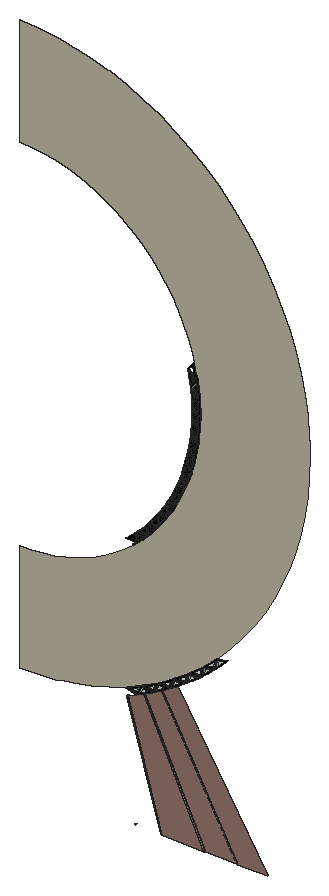
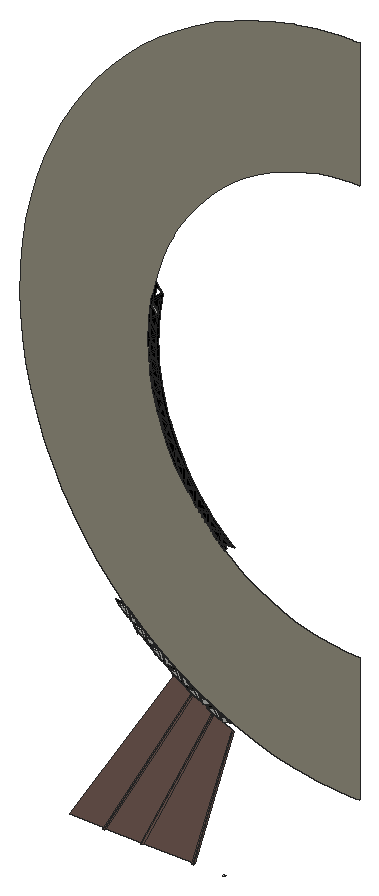
# SketchUp Ruby script. Lengths in inches.
U = 1.inch
M = Sketchup.active_model
def pt(a) = Geom::Point3d.new(a.map { |v| v * U })
def face(e, loops, mat)
  f = e.add_face(loops[0].map { |a| pt(a) })
  loops[1..].each { |l| e.add_face(l.map { |a| pt(a) }).erase! }
  f.material = f.back_material = mat if mat
  f
end
# faces: each face lists its corners as indices into pts; further lists are holes
def faces(e, pts, list, mat = nil) = list.each { |f| face(e, (f[0].is_a?(Array) ? f : [f]).map { |l| l.map { |i| pts[i] } }, mat) }
# xy, xz, yz: faces in a plane at the given z, y or x. An outline is a flat list of corners, or four numbers for a rectangle; further outlines are holes
def ring(l) = l.size == 4 ? [[l[0], l[1]], [l[2], l[1]], [l[2], l[3]], [l[0], l[3]]] : l.each_slice(2).to_a
def flat(e, list, mat, &to3) = list.each { |f| face(e, (f[0].is_a?(Array) ? f : [f]).map { |l| ring(l).map { |u, v| to3.(u, v) } }, mat) }
def xy(e, z, list, mat = nil) = flat(e, list, mat) { |x, y| [x, y, z] }
def xz(e, y, list, mat = nil) = flat(e, list, mat) { |x, z| [x, y, z] }
def yz(e, x, list, mat = nil) = flat(e, list, mat) { |y, z| [x, y, z] }
def lines(e, pts, list) = list.each { |a, b| e.add_line(pt(pts[a]), pt(pts[b])) }
# prism: a flat outline (further loops are holes) pulled along v
def prism(e, loops, v, mat = nil)
  f = face(e, loops, mat); d = Geom::Vector3d.new(v.map { |x| x * U })
  f.pushpull(f.normal.samedirection?(d) ? d.length : -d.length)
end
def box(e, o, s, mat = nil) = prism(e, [[o, [o[0] + s[0], o[1], o[2]], [o[0] + s[0], o[1] + s[1], o[2]], [o[0], o[1] + s[1], o[2]]]], [0, 0, s[2]], mat)
def at(x, y, z, deg = 0) = Geom::Transformation.translation(pt([x, y, z])) * Geom::Transformation.rotation(ORIGIN, Z_AXIS, deg.degrees)
def axes(o, x, y, z) = Geom::Transformation.new([*x, 0, *y, 0, *z, 0, *pt(o).to_a, 1])
def part(name) = M.definitions.add(name)
# library, detail: a bought-in or finely detailed component or shape, given as its bounding box
def library(name, o, s) = part(name).tap { |d| box(d.entities, o, s) }
def detail(e, o, s) = box(e.add_group.entities, o, s)
def put(e, d, t, mat = nil) = e.add_instance(d, t).tap { |i| i.material = mat if mat }
def group(e, t, mat = nil) = e.add_group.tap { |g| g.transformation = t; g.material = mat if mat }.entities
root = M.entities
M.materials.add("Tafisa-Terrarossa-PM780-4K").color = [148, 117, 107]
M.materials.add("Uniboard-L19-Putty-4K").color = [187, 181, 160]
M.materials.add("[Color M09]").color = [0, 0, 0]
xy(root,6.709,[[112.905,138,113.026,138.157],[115.672,138,115.795,138.157],[120.336,138,120.468,138.157]])
xy(root,22.994,[[118.808,138,119.552,138.157]])
xy(root,23.244,[[119.127,138,119.823,138.157]])
xy(root,33.737,[[112.411,138,113.165,138.125]],"[Color M09]")
xy(root,35.646,[[114.454,138,115.13,138.125]],"[Color M09]")
xy(root,35.892,[[114.604,138,115.342,138.157]],"[Color M09]")
xy(root,37.097,[[115.614,138,116.248,138.157]],"[Color M09]")
xy(root,37.343,[[115.741,138,116.358,138.157]],"[Color M09]")
xy(root,38.633,[[116.62,138,117.217,138.157]],"[Color M09]")
xy(root,38.879,[[116.715,138,117.293,138.157]],"[Color M09]")
xz(root,138,[[115.795,6.709,120.336,6.709,113.927,19.441,113.923,19.447,113.124,19.101,112.216,18.708],[120.468,6.709,123.753,6.709,115.795,20.393,114.914,19.943,114.032,19.494],[123.89,6.709,127.065,6.709,117.499,21.4,116.647,20.896,115.898,20.452,123.855,6.768]],"Tafisa-Terrarossa-PM780-4K")
xz(root,138,[[[113.124,19.101,113.73,20.136,111.955,19.367],[113.062,19.243,112.356,19.404,113.429,19.869]],[[113.124,19.101,113.923,19.447,114.032,19.494,114.914,19.943,113.73,20.136],[113.425,19.368,113.795,19.998,114.516,19.881,113.979,19.607]],[[114.914,19.943,115.454,21.014,113.73,20.136],[114.843,20.082,114.128,20.198,115.17,20.729]],[[114.914,19.943,115.795,20.393,115.898,20.452,116.647,20.896,115.454,21.014],[115.198,20.229,115.527,20.881,116.254,20.809,115.735,20.502]],[[116.647,20.896,117.119,21.999,115.454,21.014],[116.568,21.03,115.847,21.101,116.853,21.696]],
  [[116.647,20.896,117.499,21.4,117.597,21.466,118.317,21.956,117.119,21.999],[116.913,21.199,117.2,21.87,117.931,21.845,117.432,21.506]],[[118.317,21.956,118.704,23.076,117.119,21.999],[118.229,22.085,117.506,22.11,118.463,22.76]],[[118.317,21.956,119.136,22.512,119.229,22.586,119.918,23.119,118.762,23.119,118.719,23.086,118.704,23.076],[118.559,22.272,118.808,22.994,119.552,22.994,119.062,22.614]],[[118.762,23.119,119.918,23.119,120.248,24.272],[119.127,23.244,120.022,23.938,119.823,23.244]],[[119.918,23.119,120.7,23.725,120.789,23.803,121.442,24.38,120.248,24.272],[120.144,23.452,120.345,24.155,121.072,24.221,120.62,23.822]],
  [[120.248,24.272,121.442,24.38,121.699,25.551],[120.618,24.431,121.495,25.204,121.339,24.496]],[[121.442,24.38,122.184,25.034,122.884,25.734,121.699,25.551],[121.646,24.727,121.803,25.441,122.525,25.552,122.099,25.126]],[[112.052,33.614,113.301,33.614,113.203,34.599,112.336,33.835],[112.411,33.737,112.415,33.74,113.104,34.348,113.165,33.737]],[[113.301,33.614,113.753,34.013,114.331,34.591,113.203,34.599],[113.399,33.865,113.339,34.475,114.036,34.47,113.669,34.103]],[[114.331,34.591,114.331,35.769,114.019,35.415,113.203,34.599],[114.208,34.715,113.498,34.72,114.109,35.331,114.208,35.444]],
  [[114.331,34.591,114.605,34.865,115.402,35.769,114.331,35.769],[114.454,34.888,114.454,35.646,115.13,35.646,114.515,34.95]],[[114.331,35.769,115.402,35.769,115.491,35.884,115.491,37.194,114.783,36.282],[114.604,35.892,114.878,36.203,115.368,36.835,115.368,35.926,115.342,35.892]],[[115.491,35.884,116.141,36.722,116.48,37.22,115.509,37.22,115.491,37.194],[115.614,36.243,115.614,37.097,116.248,37.097,116.042,36.794]],[[115.509,37.22,116.48,37.22,116.499,38.756,116.14,38.15],[115.741,37.343,116.244,38.084,116.37,38.297,116.358,37.343]],[[116.48,37.22,116.819,37.719,117.432,38.756,116.499,38.756],[116.608,37.628,116.62,38.633,117.217,38.633,116.715,37.785]],
  [[116.499,38.756,117.432,38.756,117.252,40.173,116.728,39.144],[116.715,38.879,116.836,39.084,117.181,39.761,117.293,38.879]],[[117.432,38.756,117.979,39.83,118.371,40.735,117.252,40.173],[117.504,39.168,117.385,40.102,118.124,40.473,117.868,39.883]],[[117.252,40.173,118.371,40.735,117.906,41.776,117.711,41.233],[117.5,40.435,117.825,41.187,117.919,41.447,118.211,40.792]],[[118.371,40.735,118.458,40.937,118.867,42.071,118.911,42.225,117.906,41.776],[118.367,41.046,118.069,41.714,118.71,42]],[[117.906,41.776,118.911,42.225,118.424,43.428,118.102,42.319],[118.12,42.006,118.219,42.281,118.443,43.053,118.753,42.288]],
  [[118.911,42.225,119.203,43.228,119.334,43.816,118.424,43.428],[118.892,42.6,118.584,43.362,119.162,43.609,119.084,43.259]],[[118.424,43.428,119.334,43.816,118.69,44.641,118.676,44.555],[118.597,43.635,118.757,44.354,119.139,43.867]],[[119.334,43.816,119.466,44.405,119.605,45.287,118.69,44.641],[119.271,44.097,118.866,44.615,119.438,45.018,119.345,44.428]],[[118.69,44.641,119.605,45.287,118.911,46.271,118.857,45.696],[118.857,44.909,118.979,45.68,119.002,45.928,119.434,45.316]],[[119.605,45.287,119.654,45.595,119.768,46.795,118.911,46.271],[119.531,45.605,119.087,46.234,119.622,46.562,119.532,45.611]],
  [[118.911,46.271,119.768,46.795,118.984,47.423,118.966,46.846],[119.057,46.504,119.088,46.838,119.099,47.173,119.554,46.809]],[[119.768,46.795,119.806,48,118.984,47.423],[119.653,47.045,119.189,47.416,119.675,47.758]],[[118.984,47.423,119.806,48,118.984,48.577,119.002,48],[119.114,47.665,119.125,48,119.114,48.335,119.592,48]],[119.806,48,119.768,49.205,119.761,49.281,119.637,49.281,119.645,49.197,119.675,48.242,119.156,48.607,119.637,49.281,119.761,49.281,119.728,49.621,118.984,48.577],[[118.984,48.577,119.728,49.621,118.857,50.304,118.966,49.154],[119.095,48.945,119.088,49.162,119.006,50.031,119.56,49.597]],
  [[119.728,49.621,119.654,50.405,119.533,51.168,118.857,50.304],[119.579,49.895,119.03,50.325,119.456,50.87,119.532,50.389]],[[118.857,50.304,119.533,51.168,118.55,52.008,118.676,51.445],[118.934,50.602,118.797,51.468,118.751,51.675,119.364,51.151]],[[119.533,51.168,119.466,51.595,119.203,52.772,118.55,52.008],[119.36,51.478,118.724,52.022,119.136,52.505,119.345,51.572]]],"[Color M09]")
xz(root,138.125,[[112.411,33.737,113.165,33.737,113.104,34.348,112.415,33.74],[113.399,33.865,113.669,34.103,114.036,34.47,113.339,34.475],[114.208,34.715,114.208,35.444,114.109,35.331,113.498,34.72],[114.454,34.888,114.515,34.95,115.13,35.646,114.454,35.646]],"[Color M09]")
xz(root,138.157,[[113.062,19.243,113.429,19.869,112.356,19.404],[113.425,19.368,113.979,19.607,114.516,19.881,113.795,19.998],[114.843,20.082,115.17,20.729,114.128,20.198],[115.198,20.229,115.735,20.502,116.254,20.809,115.527,20.881],[116.568,21.03,116.853,21.696,115.847,21.101],
  [116.913,21.199,117.432,21.506,117.931,21.845,117.2,21.87],[118.229,22.085,118.463,22.76,117.506,22.11],[118.559,22.272,119.062,22.614,119.552,22.994,118.808,22.994],[119.127,23.244,119.823,23.244,120.022,23.938],[120.144,23.452,120.62,23.822,121.072,24.221,120.345,24.155],
  [120.618,24.431,121.339,24.496,121.495,25.204],[121.646,24.727,122.099,25.126,122.525,25.552,121.803,25.441]])
xz(root,138.157,[[115.672,6.709,115.795,6.709,112.216,18.708,112.104,18.668],[120.336,6.709,120.468,6.709,114.032,19.494,113.923,19.447,113.927,19.441],[123.753,6.709,123.89,6.709,123.855,6.768,115.898,20.452,115.795,20.393]],"Tafisa-Terrarossa-PM780-4K")
xz(root,138.157,[[100.618,17.205,100.931,17.214,101.585,17.235,102.552,17.265,104.478,17.447,105.433,17.599,106.389,17.75,108.277,18.172,110.134,18.712,111.955,19.367,113.73,20.136,115.454,21.014,117.119,21.999,118.704,23.076,118.719,23.086,118.762,23.119,120.248,24.272,121.699,25.551,123.067,26.919,124.346,28.37,125.532,29.899,126.619,31.499,127.604,33.164,128.483,34.888,128.867,35.776,129.251,36.663,129.906,38.484,130.446,40.342,130.868,42.23,131.171,44.14,131.353,46.066,131.413,48,131.373,49.281,131.353,49.934,131.171,51.86,130.868,53.77,130.446,55.658,129.906,57.516,129.251,59.337,128.483,61.112,127.604,62.836,126.619,64.501,125.532,66.101,124.346,67.63,123.067,69.081,121.699,70.449,120.248,71.728,118.719,72.914,117.119,74.001,115.454,74.986,113.73,75.864,111.955,76.633,110.134,77.288,109.87,77.365,108.277,77.828,106.612,78.2,106.389,78.25,105.433,78.401,104.478,78.553,102.552,78.735,101.327,78.773,101.236,78.776,101.221,78.776,100.618,78.795,100.618,67.1875,101.221,67.169,101.823,67.15,103.023,67.036,104.213,66.848,105.39,66.585,106.547,66.248,107.682,65.84,108.788,65.361,109.862,64.814,110.899,64.201,111.896,63.523,112.849,62.784,113.753,61.987,114.605,61.135,115.402,60.231,116.141,59.278,116.819,58.281,117.432,57.244,117.503,57.105,117.979,56.17,118.188,55.688,118.458,55.063,118.761,54.223,118.867,53.929,119.203,52.772,119.466,51.595,119.533,51.168,119.654,50.405,119.728,49.621,119.761,49.281,119.768,49.205,119.806,48,119.768,46.795,119.654,45.595,119.605,45.287,119.466,44.405,119.334,43.816,119.203,43.228,118.911,42.225,118.867,42.071,118.458,40.937,118.371,40.735,117.979,39.83,117.432,38.756,116.819,37.719,116.48,37.22,116.141,36.722,115.491,35.884,115.402,35.769,114.605,34.865,113.753,34.013,113.301,33.614,112.849,33.216,112.052,32.598,111.939,32.51,111.896,32.477,110.899,31.799,109.862,31.186,108.788,30.639,107.682,30.16,106.547,29.752,105.39,29.415,104.213,29.152,103.023,28.964,101.823,28.85,101.221,28.831,100.618,28.8125]],"Uniboard-L19-Putty-4K")
xz(root,138.157,[[114.604,35.892,115.342,35.892,115.368,35.926,115.368,36.835,114.878,36.203],[115.614,36.243,116.042,36.794,116.248,37.097,115.614,37.097],[115.741,37.343,116.358,37.343,116.37,38.297,116.244,38.084],[116.608,37.628,116.715,37.785,117.217,38.633,116.62,38.633],[116.715,38.879,117.293,38.879,117.181,39.761,116.836,39.084],
  [117.504,39.168,117.868,39.883,118.124,40.473,117.385,40.102],[117.5,40.435,118.211,40.792,117.919,41.447,117.825,41.187],[118.367,41.046,118.71,42,118.069,41.714],[118.12,42.006,118.753,42.288,118.443,43.053,118.219,42.281],[118.892,42.6,119.084,43.259,119.162,43.609,118.584,43.362],
  [118.597,43.635,119.139,43.867,118.757,44.354],[119.271,44.097,119.345,44.428,119.438,45.018,118.866,44.615],[118.857,44.909,119.434,45.316,119.002,45.928,118.979,45.68],[119.531,45.605,119.532,45.611,119.622,46.562,119.087,46.234],[119.057,46.504,119.554,46.809,119.099,47.173,119.088,46.838],
  [119.653,47.045,119.675,47.758,119.189,47.416],[119.114,47.665,119.592,48,119.114,48.335,119.125,48],[119.675,48.242,119.645,49.197,119.637,49.281,119.156,48.607],[119.095,48.945,119.56,49.597,119.006,50.031,119.088,49.162],[119.579,49.895,119.532,50.389,119.456,50.87,119.03,50.325],
  [118.934,50.602,119.364,51.151,118.751,51.675,118.797,51.468]],"[Color M09]")
yz(root,114.208,[[138,34.715,138.125,35.444]],"[Color M09]")
yz(root,114.454,[[138,34.888,138.125,35.646]],"[Color M09]")
yz(root,115.368,[[138,35.926,138.157,36.835]],"[Color M09]")
yz(root,115.614,[[138,36.243,138.157,37.097]],"[Color M09]")
p = [[112.104,138,18.668],[115.672,138,6.709],[115.672,138.157,6.709],[112.104,138.157,18.668],[115.795,138,6.709],[112.216,138,18.708],
  [112.216,138.157,18.708],[115.795,138.157,6.709],[113.927,138,19.441],[120.336,138,6.709],[120.336,138.157,6.709],[113.927,138.157,19.441],
  [120.468,138,6.709],[114.032,138,19.494],[114.032,138.157,19.494],[120.468,138.157,6.709],[115.795,138,20.393],[123.753,138,6.709],
  [123.753,138.157,6.709],[115.795,138.157,20.393],[123.855,138,6.768],[115.898,138,20.452],[115.898,138.157,20.452],[123.855,138.157,6.768],
  [112.356,138,19.404],[113.062,138,19.243],[113.062,138.157,19.243],[112.356,138.157,19.404],[113.429,138,19.869],[113.429,138.157,19.869],
  [111.955,138,19.367],[113.73,138,20.136],[113.73,138.157,20.136],[111.955,138.157,19.367],[113.795,138,19.998],[113.425,138,19.368],
  [113.425,138.157,19.368],[113.795,138.157,19.998],[113.979,138,19.607],[113.979,138.157,19.607],[113.923,138,19.447],[113.923,138.157,19.447],
  [114.516,138,19.881],[114.516,138.157,19.881],[115.454,138,21.014],[115.454,138.157,21.014],[114.128,138,20.198],[114.843,138,20.082],
  [114.843,138.157,20.082],[114.128,138.157,20.198],[115.17,138,20.729],[115.17,138.157,20.729],[115.527,138,20.881],[115.198,138,20.229],
  [115.198,138.157,20.229],[115.527,138.157,20.881],[115.735,138,20.502],[115.735,138.157,20.502],[116.254,138,20.809],[116.254,138.157,20.809],
  [117.119,138,21.999],[117.119,138.157,21.999],[115.847,138,21.101],[116.568,138,21.03],[116.568,138.157,21.03],[115.847,138.157,21.101],
  [116.853,138,21.696],[116.853,138.157,21.696],[117.2,138,21.87],[116.913,138,21.199],[116.913,138.157,21.199],[117.2,138.157,21.87],
  [117.432,138,21.506],[117.432,138.157,21.506],[117.597,138,21.466],[117.499,138,21.4],[117.499,138.157,21.4],[117.597,138.157,21.466],
  [117.931,138,21.845],[117.931,138.157,21.845],[117.598,138,21.464],[117.598,138.157,21.464],[118.704,138,23.076],[118.704,138.157,23.076],
  [117.506,138,22.11],[118.229,138,22.085],[118.229,138.157,22.085],[117.506,138.157,22.11],[118.463,138,22.76],[118.463,138.157,22.76],
  [118.808,138,22.994],[118.559,138,22.272],[118.559,138.157,22.272],[118.808,138.157,22.994],[119.062,138,22.614],[119.062,138.157,22.614],
  [119.229,138,22.586],[119.136,138,22.512],[119.136,138.157,22.512],[119.229,138.157,22.586],[119.552,138,22.994],[119.552,138.157,22.994],
  [118.719,138,23.086],[118.719,138.157,23.086],[118.762,138,23.119],[118.762,138.157,23.119],[120.248,138,24.272],[120.248,138.157,24.272],
  [120.022,138,23.938],[119.127,138,23.244],[119.127,138.157,23.244],[120.022,138.157,23.938],[119.823,138,23.244],[119.823,138.157,23.244],
  [120.345,138,24.155],[120.144,138,23.452],[120.144,138.157,23.452],[120.345,138.157,24.155],[120.62,138,23.822],[120.62,138.157,23.822],
  [120.789,138,23.803],[120.7,138,23.725],[120.7,138.157,23.725],[120.789,138.157,23.803],[121.072,138,24.221],[121.072,138.157,24.221],
  [121.699,138,25.551],[121.699,138.157,25.551],[120.618,138,24.431],[121.339,138,24.496],[121.339,138.157,24.496],[120.618,138.157,24.431],
  [121.495,138,25.204],[121.495,138.157,25.204],[121.803,138,25.441],[121.646,138,24.727],[121.646,138.157,24.727],[121.803,138.157,25.441],
  [122.099,138,25.126],[122.099,138.157,25.126],[122.525,138,25.552],[122.525,138.157,25.552],[113.301,138,33.614],[112.849,138,33.216],
  [112.849,138.157,33.216],[113.301,138.157,33.614],[112.77,138,33.311],[112.975,138,33.491],[112.975,138.125,33.491],[112.77,138.125,33.311],
  [113.753,138,34.013],[113.753,138.157,34.013],[113.104,138,34.348],[112.415,138,33.74],[112.415,138.125,33.74],[113.104,138.125,34.348],
  [113.165,138,33.737],[113.165,138.125,33.737],[112.336,138,33.835],[113.203,138,34.599],[113.203,138.157,34.599],[112.336,138.157,33.835],
  [113.339,138,34.475],[113.399,138,33.865],[113.399,138.125,33.865],[113.339,138.125,34.475],[113.669,138,34.103],[113.669,138.125,34.103],
  [114.331,138,34.591],[114.331,138.157,34.591],[114.036,138,34.47],[114.036,138.125,34.47],[114.019,138,35.415],[114.019,138.157,35.415],
  [114.605,138,34.865],[114.605,138.157,34.865],[114.109,138,35.331],[113.498,138,34.72],[113.498,138.125,34.72],[114.109,138.125,35.331],
  [114.208,138,34.715],[114.208,138.125,34.715],[114.454,138,34.888],[114.515,138,34.95],[114.515,138.125,34.95],[114.454,138.125,34.888],
  [115.13,138,35.646],[115.13,138.125,35.646],[115.402,138,35.769],[115.402,138.157,35.769],[114.208,138,35.444],[114.208,138.125,35.444],
  [114.331,138,35.769],[114.331,138.157,35.769],[114.783,138,36.282],[114.783,138.157,36.282],[115.491,138,35.884],[115.491,138.157,35.884],
  [114.878,138,36.203],[114.604,138,35.892],[114.604,138.157,35.892],[114.878,138.157,36.203],[115.342,138,35.892],[115.368,138,35.926],
  [115.368,138.157,35.926],[115.342,138.157,35.892],[116.141,138,36.722],[116.141,138.157,36.722],[115.368,138,36.835],[115.368,138.157,36.835],
  [115.614,138,36.243],[116.042,138,36.794],[116.042,138.157,36.794],[115.614,138.157,36.243],[115.491,138,37.194],[115.491,138.157,37.194],
  [116.48,138,37.22],[116.48,138.157,37.22],[116.248,138,37.097],[116.248,138.157,37.097],[115.509,138,37.22],[115.509,138.157,37.22],
  [116.14,138,38.15],[116.14,138.157,38.15],[116.819,138,37.719],[116.819,138.157,37.719],[116.244,138,38.084],[115.741,138,37.343],
  [115.741,138.157,37.343],[116.244,138.157,38.084],[116.358,138,37.343],[116.37,138,38.297],[116.37,138.157,38.297],[116.358,138.157,37.343],
  [116.62,138,38.633],[116.608,138,37.628],[116.608,138.157,37.628],[116.62,138.157,38.633],[116.715,138,37.785],[116.715,138.157,37.785],
  [117.432,138,38.756],[117.432,138.157,38.756],[117.217,138,38.633],[117.217,138.157,38.633],[116.499,138,38.756],[116.499,138.157,38.756],
  [116.728,138,39.144],[116.728,138.157,39.144],[117.979,138,39.83],[117.979,138.157,39.83],[116.836,138,39.084],[116.715,138,38.879],
  [116.715,138.157,38.879],[116.836,138.157,39.084],[117.293,138,38.879],[117.181,138,39.761],[117.181,138.157,39.761],[117.293,138.157,38.879],
  [117.252,138,40.173],[117.252,138.157,40.173],[117.385,138,40.102],[117.504,138,39.168],[117.504,138.157,39.168],[117.385,138.157,40.102],
  [117.868,138,39.883],[117.868,138.157,39.883],[118.371,138,40.735],[118.371,138.157,40.735],[118.124,138,40.473],[118.124,138.157,40.473],
  [117.711,138,41.233],[117.711,138.157,41.233],[117.825,138,41.187],[117.5,138,40.435],[117.5,138.157,40.435],[117.825,138.157,41.187],
  [118.211,138,40.792],[118.211,138.157,40.792],[118.458,138,40.937],[118.458,138.157,40.937],[117.919,138,41.447],[117.919,138.157,41.447],
  [118.867,138,42.071],[118.867,138.157,42.071],[118.069,138,41.714],[118.367,138,41.046],[118.367,138.157,41.046],[118.069,138.157,41.714],
  [118.71,138,42],[118.71,138.157,42],[117.906,138,41.776],[117.906,138.157,41.776],[118.102,138,42.319],[118.102,138.157,42.319],
  [118.219,138,42.281],[118.12,138,42.006],[118.12,138.157,42.006],[118.219,138.157,42.281],[118.753,138,42.288],[118.753,138.157,42.288],
  [118.911,138,42.225],[118.911,138.157,42.225],[119.203,138,43.228],[119.203,138.157,43.228],[118.424,138,43.428],[118.424,138.157,43.428],
  [118.443,138,43.053],[118.443,138.157,43.053],[118.584,138,43.362],[118.892,138,42.6],[118.892,138.157,42.6],[118.584,138.157,43.362],
  [119.084,138,43.259],[119.084,138.157,43.259],[119.334,138,43.816],[119.334,138.157,43.816],[119.162,138,43.609],[119.162,138.157,43.609],
  [118.676,138,44.555],[118.676,138.157,44.555],[118.757,138,44.354],[118.597,138,43.635],[118.597,138.157,43.635],[118.757,138.157,44.354],
  [119.139,138,43.867],[119.139,138.157,43.867],[119.466,138,44.405],[119.466,138.157,44.405],[118.866,138,44.615],[119.271,138,44.097],
  [119.271,138.157,44.097],[118.866,138.157,44.615],[119.345,138,44.428],[119.345,138.157,44.428],[119.438,138,45.018],[119.438,138.157,45.018],
  [119.605,138,45.287],[119.605,138.157,45.287],[118.69,138,44.641],[118.69,138.157,44.641],[118.857,138,45.696],[118.857,138.157,45.696],
  [118.979,138,45.68],[118.857,138,44.909],[118.857,138.157,44.909],[118.979,138.157,45.68],[119.434,138,45.316],[119.434,138.157,45.316],
  [119.002,138,45.928],[119.002,138.157,45.928],[119.654,138,45.595],[119.654,138.157,45.595],[119.087,138,46.234],[119.531,138,45.605],
  [119.531,138.157,45.605],[119.087,138.157,46.234],[119.532,138,45.611],[119.532,138.157,45.611],[119.622,138,46.562],[119.622,138.157,46.562],
  [119.768,138,46.795],[119.768,138.157,46.795],[118.911,138,46.271],[118.911,138.157,46.271],[118.966,138,46.846],[118.966,138.157,46.846],
  [119.088,138,46.838],[119.057,138,46.504],[119.057,138.157,46.504],[119.088,138.157,46.838],[119.554,138,46.809],[119.554,138.157,46.809],
  [118.984,138,47.423],[118.984,138.157,47.423],[119.099,138,47.173],[119.099,138.157,47.173],[119.806,138,48],[119.806,138.157,48],
  [119.189,138,47.416],[119.653,138,47.045],[119.653,138.157,47.045],[119.189,138.157,47.416],[119.675,138,47.758],[119.675,138.157,47.758],
  [119.002,138,48],[119.002,138.157,48],[119.125,138,48],[119.114,138,47.665],[119.114,138.157,47.665],[119.125,138.157,48],
  [119.592,138,48],[119.592,138.157,48],[118.984,138,48.577],[118.984,138.157,48.577],[119.114,138,48.335],[119.114,138.157,48.335],
  [119.768,138,49.205],[119.768,138.157,49.205],[119.156,138,48.607],[119.675,138,48.242],[119.675,138.157,48.242],[119.156,138.157,48.607],
  [119.645,138,49.197],[119.645,138.157,49.197],[118.966,138,49.154],[118.966,138.157,49.154],[119.637,138,49.281],[119.637,138.157,49.281],
  [119.088,138,49.162],[119.095,138,48.945],[119.095,138.157,48.945],[119.088,138.157,49.162],[119.56,138,49.597],[119.56,138.157,49.597],
  [118.857,138,50.304],[118.857,138.157,50.304],[119.006,138,50.031],[119.006,138.157,50.031],[119.761,138,49.281],[119.761,138.157,49.281],
  [119.728,138,49.621],[119.728,138.157,49.621],[119.654,138,50.405],[119.654,138.157,50.405],[119.03,138,50.325],[119.579,138,49.895],
  [119.579,138.157,49.895],[119.03,138.157,50.325],[119.532,138,50.389],[119.532,138.157,50.389],[118.676,138,51.445],[118.676,138.157,51.445],
  [119.456,138,50.87],[119.456,138.157,50.87],[119.533,138,51.168],[119.533,138.157,51.168],[118.797,138,51.468],[118.934,138,50.602],
  [118.934,138.157,50.602],[118.797,138.157,51.468],[119.364,138,51.151],[119.364,138.157,51.151],[118.751,138,51.675],[118.751,138.157,51.675],
  [119.466,138,51.595],[119.466,138.157,51.595],[115.682,138,6.675],[112.905,138,6.709],[112.911,138,6.682],[121.25,138,48.506],
  [121.262,138,48.53]]
faces(root,p,[[0,1,2,3],[4,5,6,7],[8,9,10,11],[12,13,14,15],[16,17,18,19],[20,21,22,23]],"Tafisa-Terrarossa-PM780-4K")
faces(root,p,[[24,25,26,27],[25,28,29,26],[28,24,27,29],[34,35,36,37],[35,38,39,36],[40,8,11,41],[13,40,41,14],[38,42,43,39],
  [42,34,37,43],[46,47,48,49],[47,50,51,48],[50,46,49,51],[52,53,54,55],[53,56,57,54],[21,16,19,22],[56,58,59,57],
  [58,52,55,59],[62,63,64,65],[63,66,67,64],[66,62,65,67],[68,69,70,71],[69,72,73,70],[74,75,76,77],[72,78,79,73],
  [80,74,77,81],[78,68,71,79],[84,85,86,87],[88,84,87,89],[85,88,89,86],[90,91,92,93],[91,94,95,92],[96,97,98,99],
  [94,100,101,95],[108,109,110,111],[112,108,111,113],[114,115,116,117],[115,118,119,116],[120,121,122,123],[118,124,125,119],[124,114,117,125],
  [128,129,130,131],[132,128,131,133],[129,132,133,130],[134,135,136,137],[135,138,139,136],[140,134,137,141],[432,424,427,433],[440,442,443,441]])
faces(root,p,[[30,31,32,33],[31,44,45,32],[44,60,61,45],[60,82,83,61],[82,102,103,83],[102,104,105,103]],"Uniboard-L19-Putty-4K")
faces(root,p,[[104,106,107,105],[106,126,127,107],[142,143,144,145],[146,147,148,149],[150,142,145,151],[152,153,154,155],[156,152,155,157],[158,159,160,161],
  [162,163,164,165],[163,166,167,164],[168,150,151,169],[166,170,171,167],[170,162,165,171],[159,172,173,160],[174,168,169,175],[176,177,178,179],
  [177,180,181,178],[182,183,184,185],[183,186,187,184],[188,174,175,189],[190,176,179,191],[172,192,193,173],[192,194,195,193],[196,188,189,197],
  [198,199,200,201],[202,203,204,205],[206,196,197,207],[208,198,201,209],[210,211,212,213],[194,214,215,195],[216,206,207,217],[211,218,219,212],
  [214,220,221,215],[220,222,223,221],[224,216,217,225],[226,227,228,229],[230,231,232,233],[234,235,236,237],[235,238,239,236],[240,224,225,241],
  [238,242,243,239],[222,244,245,223],[231,226,229,232],[244,246,247,245],[248,240,241,249],[250,251,252,253],[254,255,256,257],[246,258,259,247],
  [255,250,253,256],[260,261,262,263],[261,264,265,262],[266,248,249,267],[264,268,269,265],[268,260,263,269],[258,270,271,259],[272,273,274,275],
  [273,276,277,274],[278,266,267,279],[276,280,281,277],[282,278,279,283],[284,285,286,287],[285,288,289,286],[270,290,291,271],[280,272,275,281],
  [288,284,287,289],[290,292,293,291],[294,295,296,297],[295,298,299,296],[300,282,283,301],[302,300,301,303],[292,304,305,293],[306,294,297,307],
  [298,306,307,299],[308,309,310,311],[309,312,313,310],[314,302,303,315],[312,316,317,313],[304,318,319,305],[316,308,311,317],[320,321,322,323],
  [321,324,325,322],[326,314,315,327],[324,320,323,325],[328,329,330,331],[329,332,333,330],[332,334,335,333],[336,326,327,337],[318,338,339,319],
  [338,340,341,339],[334,328,331,335],[342,343,344,345],[343,346,347,344],[346,348,349,347],[350,336,337,351],[352,353,354,355],[353,356,357,354],
  [356,358,359,357],[360,350,351,361],[340,362,363,341],[348,342,345,349],[358,352,355,359],[362,364,365,363],[366,367,368,369],[367,370,371,368],
  [364,372,373,365],[374,366,369,375],[370,374,375,371],[376,360,361,377],[378,379,380,381],[379,382,383,380],[372,384,385,373],[382,378,381,383],
  [386,387,388,389],[387,390,391,388],[384,392,393,385],[394,386,389,395],[390,394,395,391],[396,376,377,397],[398,399,400,401],[399,402,403,400],
  [392,404,405,393],[406,398,401,407],[408,409,410,411],[409,412,413,410],[404,414,415,405],[416,408,411,417],[402,406,407,403],[418,396,397,419],
  [420,418,419,421],[412,416,417,413],[422,420,421,423],[424,425,426,427],[425,428,429,426],[414,430,431,415],[428,432,433,429],[434,422,423,435],
  [436,437,438,439],[437,440,441,438],[444,434,435,445]],"[Color M09]")
lines(root,p,[[1,446],[447,448],[449,450]])
